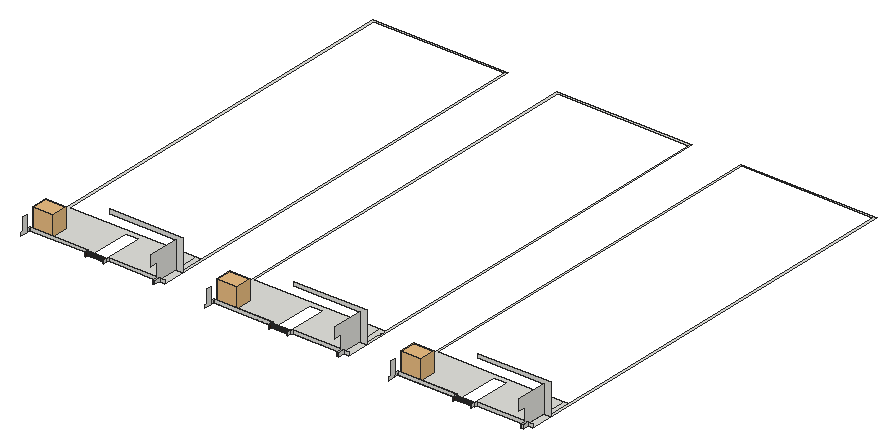
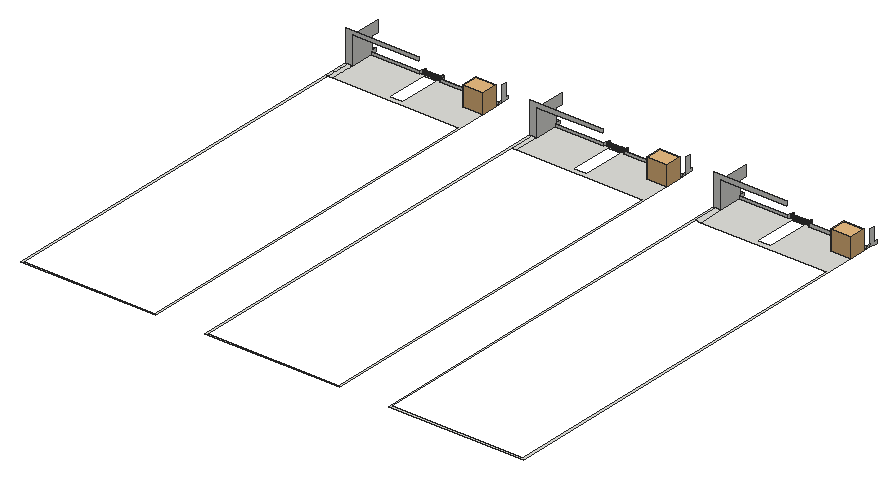
# SketchUp Ruby script. Lengths in inches.
U = 1.inch
M = Sketchup.active_model
def pt(a) = Geom::Point3d.new(a.map { |v| v * U })
def face(e, loops, mat)
  f = e.add_face(loops[0].map { |a| pt(a) })
  loops[1..].each { |l| e.add_face(l.map { |a| pt(a) }).erase! }
  f.material = f.back_material = mat if mat
  f
end
# faces: each face lists its corners as indices into pts; further lists are holes
def faces(e, pts, list, mat = nil) = list.each { |f| face(e, (f[0].is_a?(Array) ? f : [f]).map { |l| l.map { |i| pts[i] } }, mat) }
# xy, xz, yz: faces in a plane at the given z, y or x. An outline is a flat list of corners, or four numbers for a rectangle; further outlines are holes
def ring(l) = l.size == 4 ? [[l[0], l[1]], [l[2], l[1]], [l[2], l[3]], [l[0], l[3]]] : l.each_slice(2).to_a
def flat(e, list, mat, &to3) = list.each { |f| face(e, (f[0].is_a?(Array) ? f : [f]).map { |l| ring(l).map { |u, v| to3.(u, v) } }, mat) }
def xy(e, z, list, mat = nil) = flat(e, list, mat) { |x, y| [x, y, z] }
def xz(e, y, list, mat = nil) = flat(e, list, mat) { |x, z| [x, y, z] }
def yz(e, x, list, mat = nil) = flat(e, list, mat) { |y, z| [x, y, z] }
def lines(e, pts, list) = list.each { |a, b| e.add_line(pt(pts[a]), pt(pts[b])) }
# prism: a flat outline (further loops are holes) pulled along v
def prism(e, loops, v, mat = nil)
  f = face(e, loops, mat); d = Geom::Vector3d.new(v.map { |x| x * U })
  f.pushpull(f.normal.samedirection?(d) ? d.length : -d.length)
end
def box(e, o, s, mat = nil) = prism(e, [[o, [o[0] + s[0], o[1], o[2]], [o[0] + s[0], o[1] + s[1], o[2]], [o[0], o[1] + s[1], o[2]]]], [0, 0, s[2]], mat)
def at(x, y, z, deg = 0) = Geom::Transformation.translation(pt([x, y, z])) * Geom::Transformation.rotation(ORIGIN, Z_AXIS, deg.degrees)
def axes(o, x, y, z) = Geom::Transformation.new([*x, 0, *y, 0, *z, 0, *pt(o).to_a, 1])
def part(name) = M.definitions.add(name)
# library, detail: a bought-in or finely detailed component or shape, given as its bounding box
def library(name, o, s) = part(name).tap { |d| box(d.entities, o, s) }
def detail(e, o, s) = box(e.add_group.entities, o, s)
def put(e, d, t, mat = nil) = e.add_instance(d, t).tap { |i| i.material = mat if mat }
def group(e, t, mat = nil) = e.add_group.tap { |g| g.transformation = t; g.material = mat if mat }.entities
root = M.entities
M.materials.add("[Wood Veneer 01]").color = [51, 28, 15]
c1 = library("Round Planter with Plant",[-35.48,-39.77,0],[80.62,63.55,77.875])
xy(root,512.6875,[[593.5,270.05,602.25,293.45],[1327.0625,270.05,1335.8125,293.45],[2060.625,270.05,2069.375,293.45],[318.81,271.96,322.23,286.21],[1052.37,271.96,1055.8,286.21],
  [1785.93,271.96,1789.36,286.21],[390.12,272.89,393.55,286.21],[1123.68,272.89,1127.11,286.21],[1857.25,272.89,1860.67,286.21],[324.81,282.52,328.23,286.21],
  [330.81,282.52,334.23,286.21],[336.81,282.52,340.23,286.21],[342.81,282.52,346.23,286.21],[1058.37,282.52,1061.8,286.21],[1064.37,282.52,1067.8,286.21],
  [1070.37,282.52,1073.8,286.21],[1076.37,282.52,1079.8,286.21],[1791.93,282.52,1795.36,286.21],[1797.93,282.52,1801.36,286.21],[1803.93,282.52,1807.36,286.21],
  [1809.93,282.52,1813.36,286.21],[348.81,283.46,352.23,286.21],[354.81,283.46,358.23,286.21],[360.81,283.46,364.23,286.21],[366.81,283.46,370.23,286.21],
  [372.81,283.46,376.23,286.21],[378.81,283.46,382.23,286.21],[384.81,283.46,388.23,286.21],[1082.37,283.46,1085.8,286.21],[1088.37,283.46,1091.8,286.21],
  [1094.37,283.46,1097.8,286.21],[1100.37,283.46,1103.8,286.21],[1106.37,283.46,1109.8,286.21],[1112.37,283.46,1115.8,286.21],[1118.37,283.46,1121.8,286.21],
  [1815.93,283.46,1819.36,286.21],[1821.93,283.46,1825.36,286.21],[1827.93,283.46,1831.36,286.21],[1833.93,283.46,1837.36,286.21],[1839.93,283.46,1843.36,286.21],
  [1845.93,283.46,1849.36,286.21],[1851.93,283.46,1855.36,286.21],[[315.43,286.21,396.57,286.21,396.57,293.45,593.5,293.45,593.5,483.79,90.36,483.79,90.36,1996.66,614.76,1996.66,614.76,381.35,622,381.35,622,2003.89,83.125,2003.89,83.125,294.83,315.43,294.83],[328.03,293.45,382.74,465.02]],[[1049,286.21,1130.14,286.21,1130.14,293.45,1327.0625,293.45,1327.0625,483.79,823.93,483.79,823.93,1996.66,1348.32,1996.66,1348.32,381.35,1355.5625,381.35,1355.5625,2003.89,816.6875,2003.89,816.6875,294.83,1049,294.83],[1061.59,293.45,1116.3,465.02]],[[1782.56,286.21,1863.7,286.21,1863.7,293.45,2060.625,293.45,2060.625,483.79,1557.49,483.79,1557.49,1996.66,2081.89,1996.66,2081.89,381.35,2089.125,381.35,2089.125,2003.89,1550.25,2003.89,1550.25,294.83,1782.56,294.83],[1795.15,293.45,1849.87,465.02]],
  [593.5,293.45,622,381.35],[1327.0625,293.45,1355.5625,381.35],[2060.625,293.45,2089.125,381.35],[83.125,293.46,90.36,294.83],[90.36,293.46,315.43,294.83],
  [816.6875,293.46,823.93,294.83],[823.93,293.46,1049,294.83],[1550.25,293.46,1557.49,294.83],[1557.49,293.46,1782.56,294.83],[593.5,381.35,614.76,483.79],
  [1327.0625,381.35,1348.32,483.79],[2060.625,381.35,2081.89,483.79]])
xz(root,270.05,[[593.5,512.6875,602.25,524.9375],[1327.0625,512.6875,1335.8125,524.9375],[2060.625,512.6875,2069.375,524.9375]])
xz(root,271.96,[[318.81,512.6875,322.23,524.9375],[1052.37,512.6875,1055.8,524.9375],[1785.93,512.6875,1789.36,524.9375]],"[Wood Veneer 01]")
xz(root,272.89,[[390.12,512.6875,393.55,524.9375],[1123.68,512.6875,1127.11,524.9375],[1857.25,512.6875,1860.67,524.9375]])
xz(root,282.52,[[324.81,512.6875,328.23,524.9375],[330.81,512.6875,334.23,524.9375],[336.81,512.6875,340.23,524.9375],[342.81,512.6875,346.23,524.9375],[1058.37,512.6875,1061.8,524.9375],
  [1064.37,512.6875,1067.8,524.9375],[1070.37,512.6875,1073.8,524.9375],[1076.37,512.6875,1079.8,524.9375],[1791.93,512.6875,1795.36,524.9375],[1797.93,512.6875,1801.36,524.9375],
  [1803.93,512.6875,1807.36,524.9375],[1809.93,512.6875,1813.36,524.9375]],"[Wood Veneer 01]")
xz(root,283.46,[[348.81,512.6875,352.23,524.9375],[354.81,512.6875,358.23,524.9375],[360.81,512.6875,364.23,524.9375],[366.81,512.6875,370.23,524.9375],[372.81,512.6875,376.23,524.9375],
  [378.81,512.6875,382.23,524.9375],[384.81,512.6875,388.23,524.9375],[1082.37,512.6875,1085.8,524.9375],[1088.37,512.6875,1091.8,524.9375],[1094.37,512.6875,1097.8,524.9375],
  [1100.37,512.6875,1103.8,524.9375],[1106.37,512.6875,1109.8,524.9375],[1112.37,512.6875,1115.8,524.9375],[1118.37,512.6875,1121.8,524.9375],[1815.93,512.6875,1819.36,524.9375],
  [1821.93,512.6875,1825.36,524.9375],[1827.93,512.6875,1831.36,524.9375],[1833.93,512.6875,1837.36,524.9375],[1839.93,512.6875,1843.36,524.9375],[1845.93,512.6875,1849.36,524.9375],
  [1851.93,512.6875,1855.36,524.9375]],"[Wood Veneer 01]")
xz(root,286.21,[[315.43,512.6875,318.81,524.9375],[382.23,512.6875,384.81,524.9375],[393.55,512.6875,393.95,524.9375],[393.95,512.6875,396.57,524.9375],[1049,512.6875,1052.37,524.9375],
  [1115.8,512.6875,1118.37,524.9375],[1127.11,512.6875,1127.51,524.9375],[1127.51,512.6875,1130.14,524.9375],[1782.56,512.6875,1785.93,524.9375],[1849.36,512.6875,1851.93,524.9375],
  [1860.67,512.6875,1861.07,524.9375],[1861.07,512.6875,1863.7,524.9375]])
xz(root,286.21,[[322.23,512.6875,324.81,524.9375],[328.23,512.6875,330.81,524.9375],[334.23,512.6875,336.81,524.9375],[340.23,512.6875,342.81,524.9375],[346.23,512.6875,348.81,524.9375],
  [352.23,512.6875,354.81,524.9375],[358.23,512.6875,360.81,524.9375],[364.23,512.6875,366.81,524.9375],[370.23,512.6875,372.81,524.9375],[376.23,512.6875,378.81,524.9375],
  [388.23,512.6875,390.12,524.9375],[1055.8,512.6875,1058.37,524.9375],[1061.8,512.6875,1064.37,524.9375],[1067.8,512.6875,1070.37,524.9375],[1073.8,512.6875,1076.37,524.9375],
  [1079.8,512.6875,1082.37,524.9375],[1085.8,512.6875,1088.37,524.9375],[1091.8,512.6875,1094.37,524.9375],[1097.8,512.6875,1100.37,524.9375],[1103.8,512.6875,1106.37,524.9375],
  [1109.8,512.6875,1112.37,524.9375],[1121.8,512.6875,1123.68,524.9375],[1789.36,512.6875,1791.93,524.9375],[1795.36,512.6875,1797.93,524.9375],[1801.36,512.6875,1803.93,524.9375],
  [1807.36,512.6875,1809.93,524.9375],[1813.36,512.6875,1815.93,524.9375],[1819.36,512.6875,1821.93,524.9375],[1825.36,512.6875,1827.93,524.9375],[1831.36,512.6875,1833.93,524.9375],
  [1837.36,512.6875,1839.93,524.9375],[1843.36,512.6875,1845.93,524.9375],[1855.36,512.6875,1857.25,524.9375]],"[Wood Veneer 01]")
xz(root,293.45,[[396.57,512.6875,602.25,524.9375],[602.25,512.6875,622,524.9375],[1130.14,512.6875,1335.8125,524.9375],[1335.8125,512.6875,1355.5625,524.9375],[1863.7,512.6875,2069.375,524.9375],
  [2069.375,512.6875,2089.125,524.9375]])
xz(root,293.46,[[83.125,512.6875,315.43,524.9375],[816.6875,512.6875,1049,524.9375],[1550.25,512.6875,1782.56,524.9375]])
xz(root,294.83,[[83.125,512.6875,315.43,524.9375],[816.6875,512.6875,1049,524.9375],[1550.25,512.6875,1782.56,524.9375]])
xz(root,381.35,[[593.5,512.6875,593.5,620.22,330.81,620.22,330.81,636.53,622,636.53,622,512.6875],[1327.0625,512.6875,1327.0625,620.22,1064.37,620.22,1064.37,636.53,1355.5625,636.53,1355.5625,512.6875],[2060.625,512.6875,2060.625,620.22,1797.93,620.22,1797.93,636.53,2089.125,636.53,2089.125,512.6875]])
yz(root,83.125,[[246.64,512.6875,246.64,524.9375,258.35,524.9375,258.35,576.8125,277.39,576.8125,277.39,512.6875],[277.39,512.6875,293.46,524.9375],[293.46,512.6875,294.83,524.9375]])
yz(root,315.43,[[286.21,512.6875,293.45,524.9375],[293.45,512.6875,293.46,524.9375],[293.46,512.6875,294.83,524.9375]])
yz(root,318.81,[[271.96,512.6875,277.39,524.9375],[277.39,512.6875,286.21,524.9375]])
yz(root,322.23,[[271.96,512.6875,286.21,524.9375]],"[Wood Veneer 01]")
yz(root,324.81,[[282.52,512.6875,286.21,524.9375]])
yz(root,328.23,[[282.52,512.6875,286.21,524.9375]])
yz(root,330.81,[[282.52,512.6875,286.21,524.9375]])
yz(root,334.23,[[282.52,512.6875,286.21,524.9375]])
yz(root,336.81,[[282.52,512.6875,286.21,524.9375]])
yz(root,340.23,[[282.52,512.6875,286.21,524.9375]])
yz(root,342.81,[[282.52,512.6875,286.21,524.9375]])
yz(root,346.23,[[282.52,512.6875,286.21,524.9375]])
yz(root,348.81,[[283.46,512.6875,286.21,524.9375]])
yz(root,352.23,[[283.46,512.6875,286.21,524.9375]])
yz(root,354.81,[[283.46,512.6875,286.21,524.9375]])
yz(root,358.23,[[283.46,512.6875,286.21,524.9375]])
yz(root,360.81,[[283.46,512.6875,286.21,524.9375]])
yz(root,364.23,[[283.46,512.6875,286.21,524.9375]])
yz(root,366.81,[[283.46,512.6875,286.21,524.9375]])
yz(root,370.23,[[283.46,512.6875,286.21,524.9375]])
yz(root,372.81,[[283.46,512.6875,286.21,524.9375]])
yz(root,376.23,[[283.46,512.6875,286.21,524.9375]])
yz(root,378.81,[[283.46,512.6875,286.21,524.9375]])
yz(root,382.23,[[283.46,512.6875,286.21,524.9375]])
yz(root,384.81,[[283.46,512.6875,286.21,524.9375]])
yz(root,388.23,[[283.46,512.6875,286.21,524.9375]])
yz(root,390.12,[[272.89,512.6875,286.21,524.9375]],"[Wood Veneer 01]")
yz(root,393.55,[[272.89,512.6875,286.21,524.9375]])
yz(root,396.57,[[286.21,512.6875,293.45,524.9375]])
yz(root,593.5,[[270.05,512.6875,270.05,524.9375,289.27,524.9375,289.27,576.8125,258.35,576.8125,258.35,620.22,381.35,620.22,381.35,512.6875]])
yz(root,602.25,[[270.05,512.6875,293.45,524.9375]])
yz(root,816.6875,[[246.64,512.6875,246.64,524.9375,258.35,524.9375,258.35,576.8125,277.39,576.8125,277.39,512.6875],[277.39,512.6875,293.46,524.9375],[293.46,512.6875,294.83,524.9375]])
yz(root,1049,[[286.21,512.6875,293.45,524.9375],[293.45,512.6875,293.46,524.9375],[293.46,512.6875,294.83,524.9375]])
yz(root,1052.37,[[271.96,512.6875,277.39,524.9375],[277.39,512.6875,286.21,524.9375]])
yz(root,1055.8,[[271.96,512.6875,286.21,524.9375]],"[Wood Veneer 01]")
yz(root,1058.37,[[282.52,512.6875,286.21,524.9375]])
yz(root,1061.8,[[282.52,512.6875,286.21,524.9375]])
yz(root,1064.37,[[282.52,512.6875,286.21,524.9375]])
yz(root,1067.8,[[282.52,512.6875,286.21,524.9375]])
yz(root,1070.37,[[282.52,512.6875,286.21,524.9375]])
yz(root,1073.8,[[282.52,512.6875,286.21,524.9375]])
yz(root,1076.37,[[282.52,512.6875,286.21,524.9375]])
yz(root,1079.8,[[282.52,512.6875,286.21,524.9375]])
yz(root,1082.37,[[283.46,512.6875,286.21,524.9375]])
yz(root,1085.8,[[283.46,512.6875,286.21,524.9375]])
yz(root,1088.37,[[283.46,512.6875,286.21,524.9375]])
yz(root,1091.8,[[283.46,512.6875,286.21,524.9375]])
yz(root,1094.37,[[283.46,512.6875,286.21,524.9375]])
yz(root,1097.8,[[283.46,512.6875,286.21,524.9375]])
yz(root,1100.37,[[283.46,512.6875,286.21,524.9375]])
yz(root,1103.8,[[283.46,512.6875,286.21,524.9375]])
yz(root,1106.37,[[283.46,512.6875,286.21,524.9375]])
yz(root,1109.8,[[283.46,512.6875,286.21,524.9375]])
yz(root,1112.37,[[283.46,512.6875,286.21,524.9375]])
yz(root,1115.8,[[283.46,512.6875,286.21,524.9375]])
yz(root,1118.37,[[283.46,512.6875,286.21,524.9375]])
yz(root,1121.8,[[283.46,512.6875,286.21,524.9375]])
yz(root,1123.68,[[272.89,512.6875,286.21,524.9375]],"[Wood Veneer 01]")
yz(root,1127.11,[[272.89,512.6875,286.21,524.9375]])
yz(root,1130.14,[[286.21,512.6875,293.45,524.9375]])
yz(root,1327.0625,[[270.05,512.6875,270.05,524.9375,289.27,524.9375,289.27,576.8125,258.35,576.8125,258.35,620.22,381.35,620.22,381.35,512.6875]])
yz(root,1335.8125,[[270.05,512.6875,293.45,524.9375]])
yz(root,1550.25,[[246.64,512.6875,246.64,524.9375,258.35,524.9375,258.35,576.8125,277.39,576.8125,277.39,512.6875],[277.39,512.6875,293.46,524.9375],[293.46,512.6875,294.83,524.9375]])
yz(root,1782.56,[[286.21,512.6875,293.45,524.9375],[293.45,512.6875,293.46,524.9375],[293.46,512.6875,294.83,524.9375]])
yz(root,1785.93,[[271.96,512.6875,277.39,524.9375],[277.39,512.6875,286.21,524.9375]])
yz(root,1789.36,[[271.96,512.6875,286.21,524.9375]],"[Wood Veneer 01]")
yz(root,1791.93,[[282.52,512.6875,286.21,524.9375]])
yz(root,1795.36,[[282.52,512.6875,286.21,524.9375]])
yz(root,1797.93,[[282.52,512.6875,286.21,524.9375]])
yz(root,1801.36,[[282.52,512.6875,286.21,524.9375]])
yz(root,1803.93,[[282.52,512.6875,286.21,524.9375]])
yz(root,1807.36,[[282.52,512.6875,286.21,524.9375]])
yz(root,1809.93,[[282.52,512.6875,286.21,524.9375]])
yz(root,1813.36,[[282.52,512.6875,286.21,524.9375]])
yz(root,1815.93,[[283.46,512.6875,286.21,524.9375]])
yz(root,1819.36,[[283.46,512.6875,286.21,524.9375]])
yz(root,1821.93,[[283.46,512.6875,286.21,524.9375]])
yz(root,1825.36,[[283.46,512.6875,286.21,524.9375]])
yz(root,1827.93,[[283.46,512.6875,286.21,524.9375]])
yz(root,1831.36,[[283.46,512.6875,286.21,524.9375]])
yz(root,1833.93,[[283.46,512.6875,286.21,524.9375]])
yz(root,1837.36,[[283.46,512.6875,286.21,524.9375]])
yz(root,1839.93,[[283.46,512.6875,286.21,524.9375]])
yz(root,1843.36,[[283.46,512.6875,286.21,524.9375]])
yz(root,1845.93,[[283.46,512.6875,286.21,524.9375]])
yz(root,1849.36,[[283.46,512.6875,286.21,524.9375]])
yz(root,1851.93,[[283.46,512.6875,286.21,524.9375]])
yz(root,1855.36,[[283.46,512.6875,286.21,524.9375]])
yz(root,1857.25,[[272.89,512.6875,286.21,524.9375]],"[Wood Veneer 01]")
yz(root,1860.67,[[272.89,512.6875,286.21,524.9375]])
yz(root,1863.7,[[286.21,512.6875,293.45,524.9375]])
yz(root,2060.625,[[270.05,512.6875,270.05,524.9375,289.27,524.9375,289.27,576.8125,258.35,576.8125,258.35,620.22,381.35,620.22,381.35,512.6875]])
yz(root,2069.375,[[270.05,512.6875,293.45,524.9375]])
put(root,c1,at(852.17,348.01,512.6875))
put(root,c1,at(1585.73,348.01,512.6875))
put(root,c1,at(118.61,348.01,512.6875))
